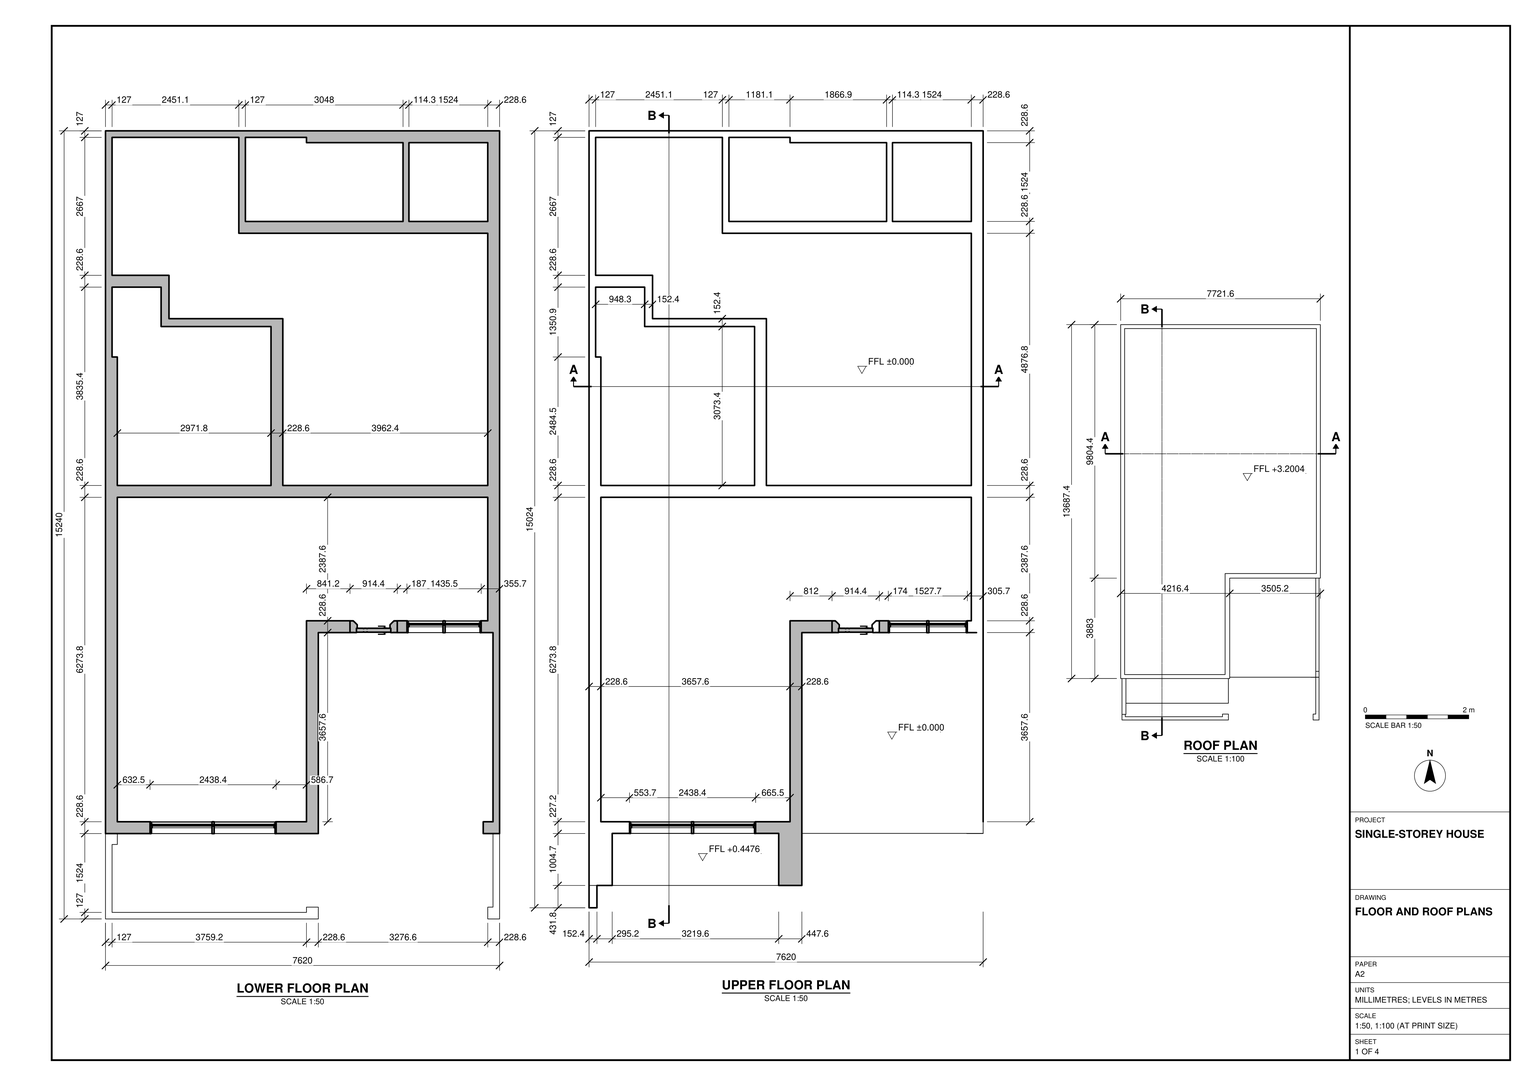
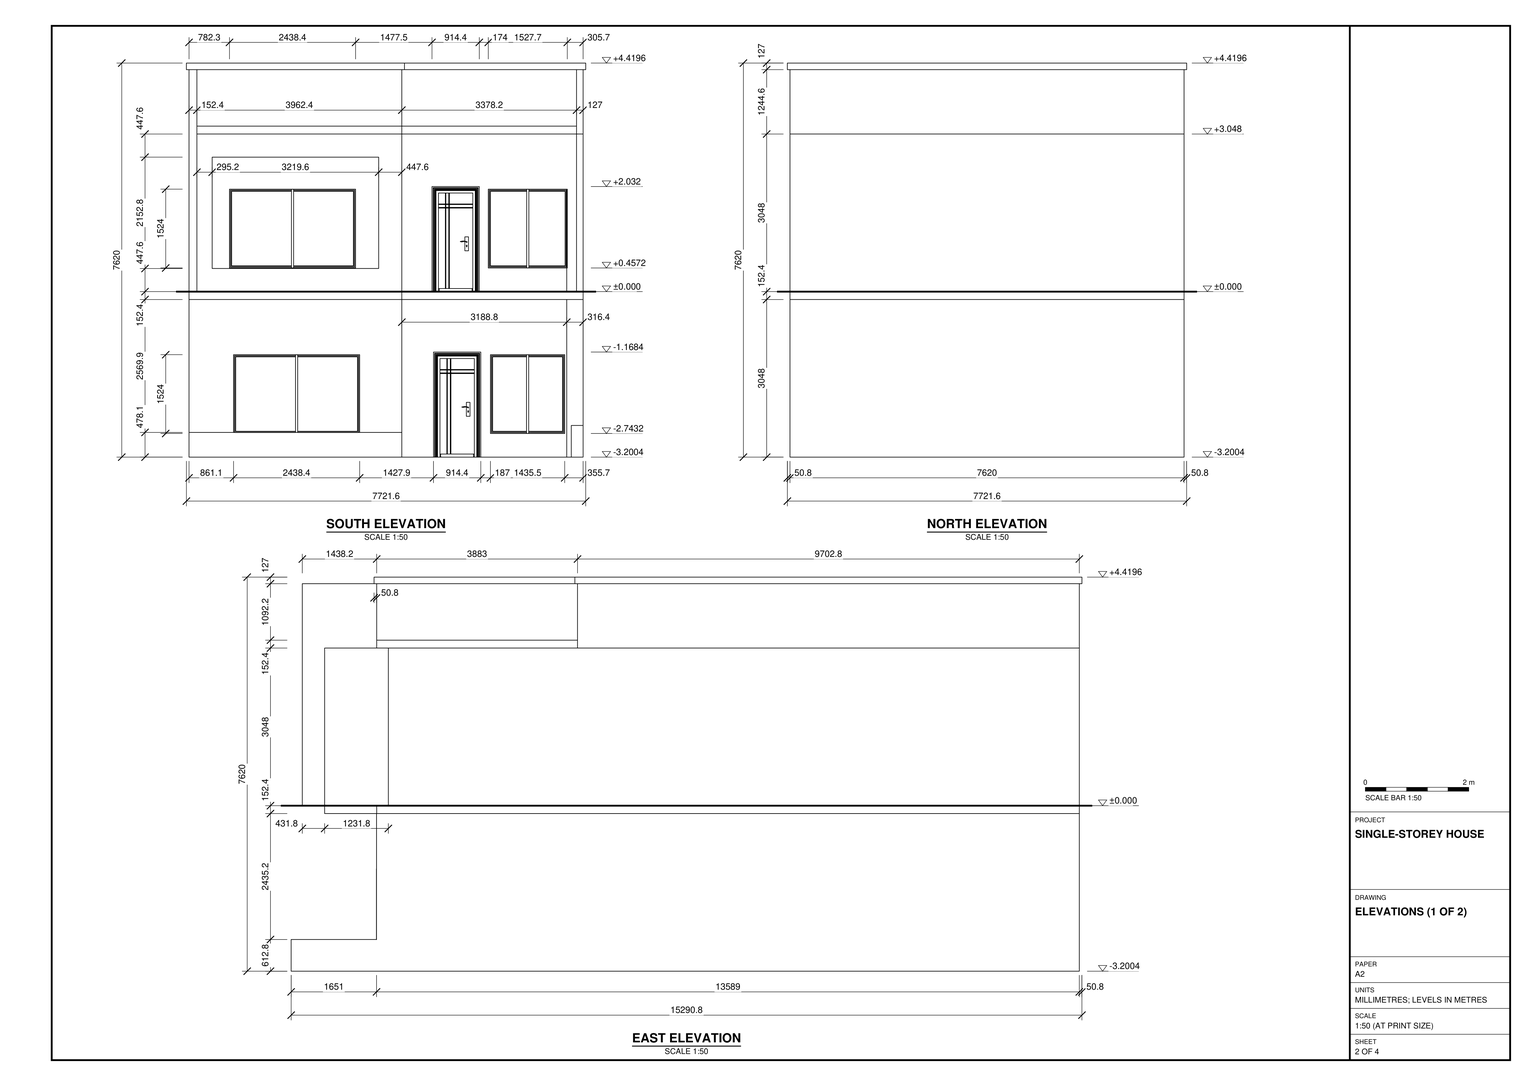
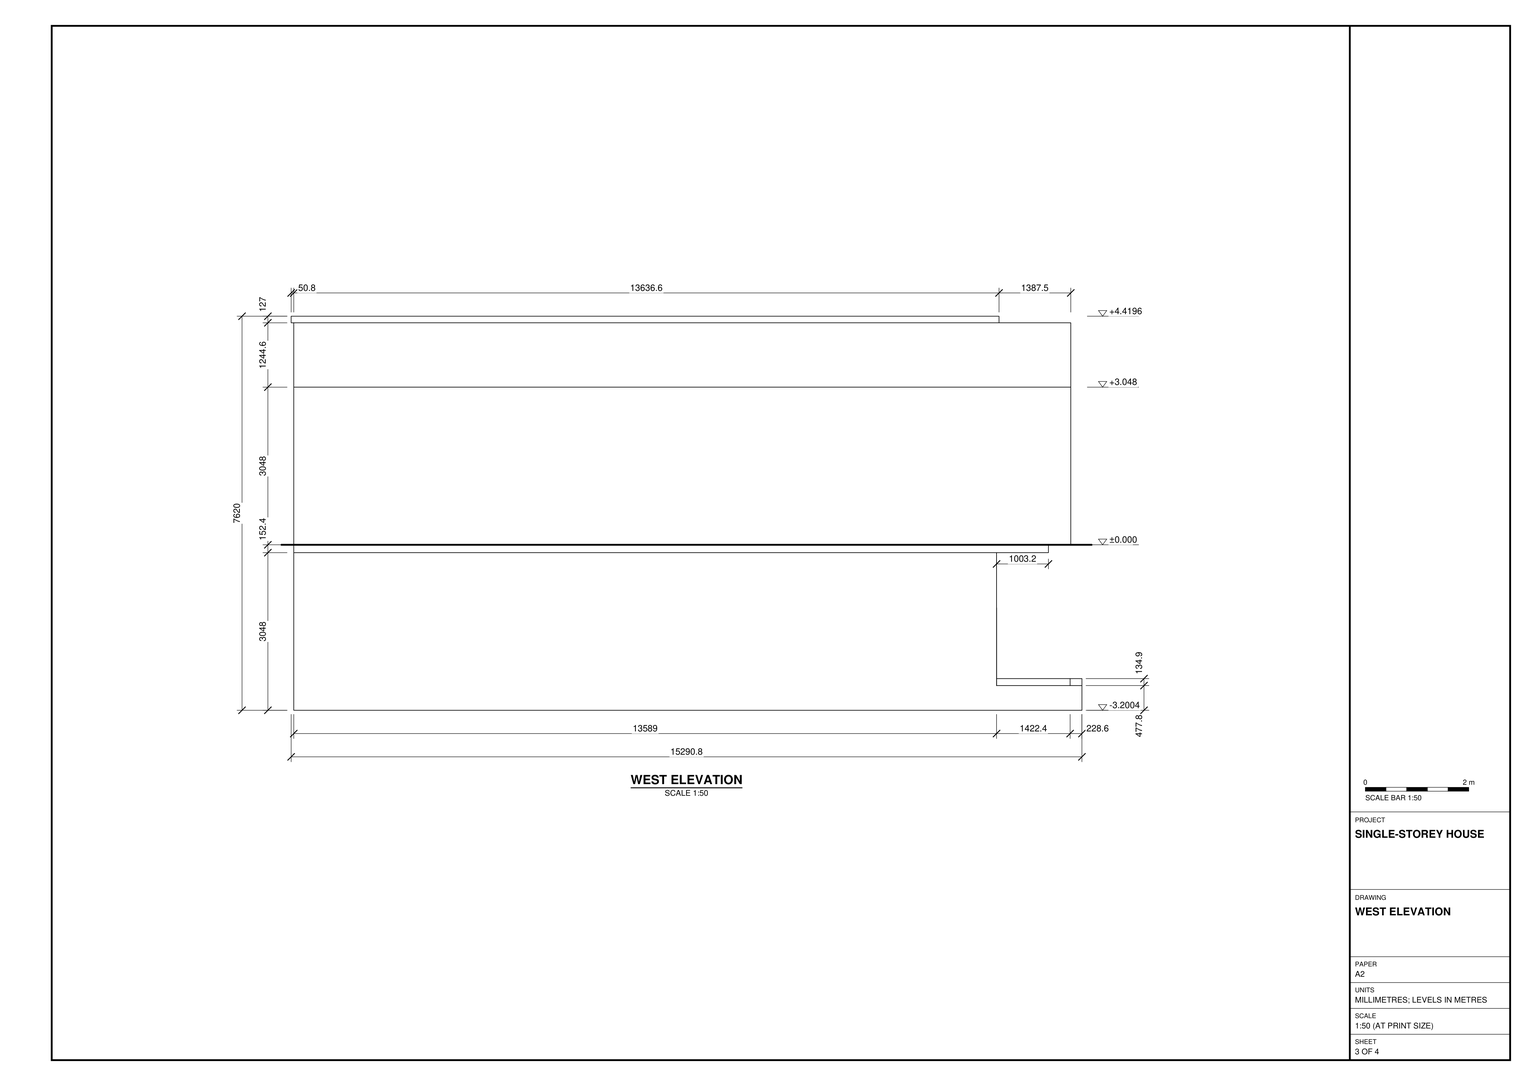
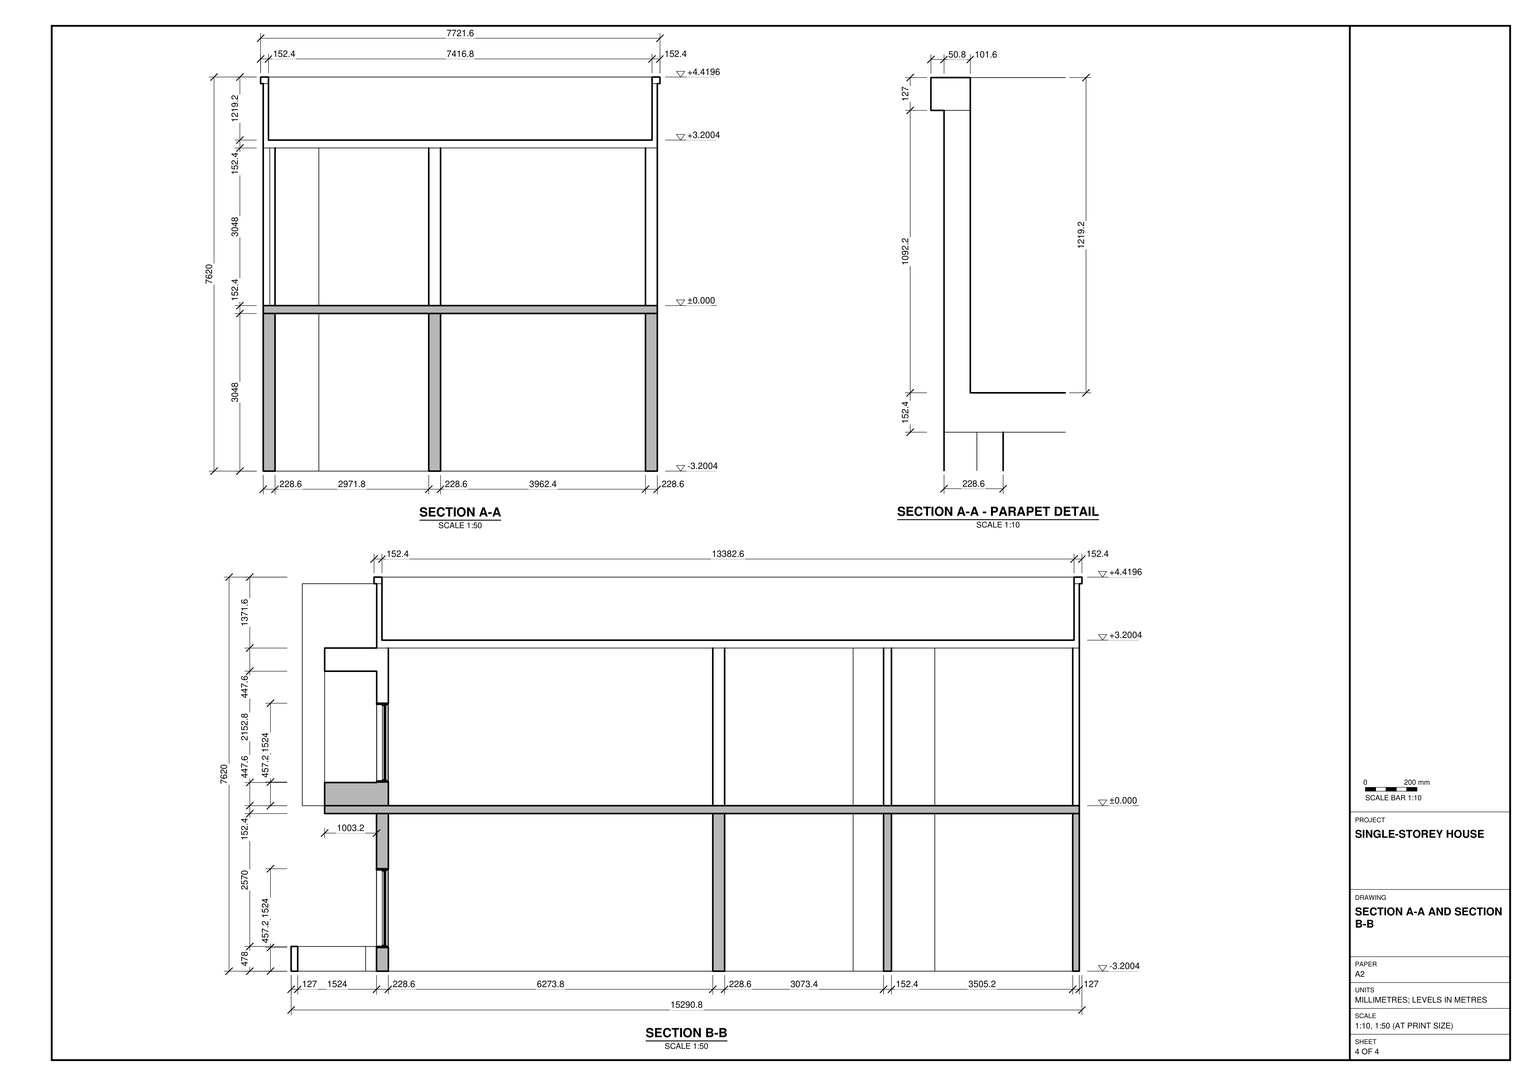
Build the house in SketchUp from task_files/diagram_01.pdf. Work in millimetres, with X running east–west and Y running north–south. The overall dimensions are 7721.6 mm wide, 15290.8 mm deep and 7620 mm high. Use the upper floor at 0 mm as the reference datum. The lower floor is at −3200.4 mm and the top of the roof edge is at +4419.6 mm.

Follow the lower and upper plans separately. At the south end, project the wide window bay forward on the west and set the entrance wall back on the east. Include the low walls and slab edges that extend beyond the enclosed rooms. Lay out the full-width cross wall, the stepped partition on the west and the smaller compartments at the north end. Use the wall thickness dimensioned for each run rather than one thickness throughout.

Fit the framed doors and divided windows on the south elevation. Keep the north, east and west faces closed as drawn. Match the flat roof to its stepped plan and show its narrow projecting cap. Keep walls, slabs, roof and any furniture or joinery pieces in separate groups or components, and use components for repeated parts. Any decor or loose items shown may be represented by suitable library components. Save one SketchUp model as output_files/flat_roofed_house_with_a_stepped_south_frontage.skp.

# SketchUp Ruby script. Lengths in millimetres.
U = 1.mm
M = Sketchup.active_model
def pt(a) = Geom::Point3d.new(a.map { |v| v * U })
def face(e, loops, mat)
  f = e.add_face(loops[0].map { |a| pt(a) })
  loops[1..].each { |l| e.add_face(l.map { |a| pt(a) }).erase! }
  f.material = f.back_material = mat if mat
  f
end
# faces: each face lists its corners as indices into pts; further lists are holes
def faces(e, pts, list, mat = nil) = list.each { |f| face(e, (f[0].is_a?(Array) ? f : [f]).map { |l| l.map { |i| pts[i] } }, mat) }
# xy, xz, yz: faces in a plane at the given z, y or x. An outline is a flat list of corners, or four numbers for a rectangle; further outlines are holes
def ring(l) = l.size == 4 ? [[l[0], l[1]], [l[2], l[1]], [l[2], l[3]], [l[0], l[3]]] : l.each_slice(2).to_a
def flat(e, list, mat, &to3) = list.each { |f| face(e, (f[0].is_a?(Array) ? f : [f]).map { |l| ring(l).map { |u, v| to3.(u, v) } }, mat) }
def xy(e, z, list, mat = nil) = flat(e, list, mat) { |x, y| [x, y, z] }
def xz(e, y, list, mat = nil) = flat(e, list, mat) { |x, z| [x, y, z] }
def yz(e, x, list, mat = nil) = flat(e, list, mat) { |y, z| [x, y, z] }
def lines(e, pts, list) = list.each { |a, b| e.add_line(pt(pts[a]), pt(pts[b])) }
# prism: a flat outline (further loops are holes) pulled along v
def prism(e, loops, v, mat = nil)
  f = face(e, loops, mat); d = Geom::Vector3d.new(v.map { |x| x * U })
  f.pushpull(f.normal.samedirection?(d) ? d.length : -d.length)
end
def box(e, o, s, mat = nil) = prism(e, [[o, [o[0] + s[0], o[1], o[2]], [o[0] + s[0], o[1] + s[1], o[2]], [o[0], o[1] + s[1], o[2]]]], [0, 0, s[2]], mat)
def at(x, y, z, deg = 0) = Geom::Transformation.translation(pt([x, y, z])) * Geom::Transformation.rotation(ORIGIN, Z_AXIS, deg.degrees)
def axes(o, x, y, z) = Geom::Transformation.new([*x, 0, *y, 0, *z, 0, *pt(o).to_a, 1])
def part(name) = M.definitions.add(name)
# library, detail: a bought-in or finely detailed component or shape, given as its bounding box
def library(name, o, s) = part(name).tap { |d| box(d.entities, o, s) }
def detail(e, o, s) = box(e.add_group.entities, o, s)
def put(e, d, t, mat = nil) = e.add_instance(d, t).tap { |i| i.material = mat if mat }
def group(e, t, mat = nil) = e.add_group.tap { |g| g.transformation = t; g.material = mat if mat }.entities
root = M.entities
M.materials.add("[Metal Silver]").color = [234, 233, 238]
M.materials.add("[Translucent Glass Blue]").color = [100, 149, 237]
M.materials["[Translucent Glass Blue]"].alpha = 0.5
M.materials.add("[Wax 01]").color = [250, 213, 163]
c1 = library("Group\#5",[0,0,0],[914.4,266,2032])
c2 = part("Group12\#2")
box(c2.entities,[26,54.1,26],[2386.4,16,1472])
c3 = library("Group\#6",[0,0,0],[914.4,266,2032])
c4 = part("Group19\#2")
box(c4.entities,[26,54.9,26],[2386.4,16,1472])
c5 = part("Group22\#2")
box(c5.entities,[26,54.9,26],[1475.7,16,1472])
c6 = part("Group25\#2")
box(c6.entities,[26,54.9,26],[1383.4,16,1472])
xy(root,0,[[[50.8,0,50.8,15240,7670.8,15240,7670.8,0,7442.2,0,7442.2,228.6,7543.8,228.6,7543.8,1651,7354.4,1651,7354.4,1879.6,7543.8,1879.6,7543.8,5537.2,5692.6,5537.2,5692.6,5765.8,7442.2,5765.8,7442.2,8153.4,279.4,8153.4,279.4,1879.6,3937,1879.6,3937,5765.8,4778.2,5765.8,4778.2,5537.2,4165.6,5537.2,4165.6,1651,279.4,1651,279.4,1440.1,177.8,1440.1,177.8,127,3937,127,3937,228.6,4165.6,228.6,4165.6,0],[3479.8,8382,7442.2,8382,7442.2,13258.8,2628.9,13258.8,2628.9,15113,177.8,15113,177.8,12446,1278.5,12446,1278.5,11607.8,3479.8,11607.8],[279.4,8382,3251.2,8382,3251.2,11455.4,1126.1,11455.4,1126.1,12217.4,177.8,12217.4,177.8,10866.5,279.4,10866.5],[2755.9,13487.4,5803.9,13487.4,5803.9,15011.4,3937,15011.4,3937,15113,2755.9,15113],[5918.2,13487.4,7442.2,15011.4]]])
xy(root,457.2,[[911.9,1651,3350.3,1879.6],[5879.6,5537.2,7315.1,5765.8]])
xy(root,477.8,[[50.8,0,4165.6,0,4165.6,228.6,3937,228.6,3937,127,177.8,127,177.8,1440.1,279.4,1440.1,279.4,1651,50.8,1651]])
xy(root,612.8,[[7442.2,0,7670.8,0,7670.8,1651,7543.8,1651,7543.8,228.6,7442.2,228.6]])
xy(root,1981.2,[[911.9,1651,3350.3,1879.6],[5879.6,5537.2,7315.1,5765.8]])
xy(root,2032,[[4778.2,5537.2,5692.6,5765.8]])
xy(root,3048,[[[50.8,1651,4165.6,1651,4165.6,5537.2,7543.8,5537.2,7543.8,1879.6,7354.4,1879.6,7354.4,1651,7670.8,1651,7670.8,15240,50.8,15240],[279.4,1879.6,279.4,8153.4,7442.2,8153.4,7442.2,5765.8,3937,5765.8,3937,1879.6],[3479.8,8382,3479.8,11607.8,1278.5,11607.8,1278.5,12446,177.8,12446,177.8,15113,2628.9,15113,2628.9,13258.8,7442.2,13258.8,7442.2,8382],[279.4,8382,279.4,10866.5,177.8,10866.5,177.8,12217.4,1126.1,12217.4,1126.1,11455.4,3251.2,11455.4,3251.2,8382],[2755.9,13487.4,2755.9,15113,3937,15113,3937,15011.4,5803.9,15011.4,5803.9,13487.4],[5918.2,13487.4,7442.2,15011.4]]])
xz(root,0,[[50.8,0,4165.6,477.8],[7442.2,0,7670.8,612.8]])
xz(root,127,[[177.8,0,3937,477.8]])
xz(root,228.6,[[3937,0,4165.6,477.8],[7442.2,0,7543.8,612.8]])
xz(root,1440.1,[[177.8,0,279.4,477.8]])
xz(root,1651,[[[279.4,0,4165.6,0,4165.6,3048,50.8,3048,50.8,477.8,279.4,477.8],[911.9,457.2,3350.3,1981.2]],[7354.4,0,7543.8,0,7543.8,612.8,7670.8,612.8,7670.8,3048,7354.4,3048]])
xz(root,1879.6,[[[279.4,0,3937,3048],[911.9,457.2,3350.3,1981.2]],[7354.4,0,7543.8,3048]])
xz(root,5537.2,[[[4165.6,0,4778.2,0,4778.2,2032,5692.6,2032,5692.6,0,7543.8,0,7543.8,3048,4165.6,3048],[5879.6,457.2,7315.1,1981.2]]])
xz(root,5765.8,[[[3937,0,3937,3048,7442.2,3048,7442.2,0,5692.6,0,5692.6,2032,4778.2,2032,4778.2,0],[5879.6,457.2,7315.1,1981.2]]])
xz(root,8153.4,[[279.4,0,7442.2,3048]])
xz(root,8382,[[279.4,0,3251.2,3048],[3479.8,0,7442.2,3048]])
xz(root,10866.5,[[177.8,0,279.4,3048]])
xz(root,11455.4,[[1126.1,0,3251.2,3048]])
xz(root,11607.8,[[1278.5,0,3479.8,3048]])
xz(root,12217.4,[[177.8,0,1126.1,3048]])
xz(root,12446,[[177.8,0,1278.5,3048]])
xz(root,13258.8,[[2628.9,0,7442.2,3048]])
xz(root,13487.4,[[2755.9,0,5803.9,3048],[5918.2,0,7442.2,3048]])
xz(root,15011.4,[[3937,0,5803.9,3048],[5918.2,0,7442.2,3048]])
xz(root,15113,[[177.8,0,2628.9,3048],[2755.9,0,3937,3048]])
xz(root,15240,[[50.8,0,7670.8,3048]])
yz(root,50.8,[[0,0,0,477.8,1651,477.8,1651,3048,15240,3048,15240,0]])
yz(root,177.8,[[127,0,1440.1,477.8],[10866.5,0,12217.4,3048],[12446,0,15113,3048]])
yz(root,279.4,[[1440.1,0,1651,477.8],[1879.6,0,8153.4,3048],[8382,0,10866.5,3048]])
yz(root,911.9,[[1651,457.2,1879.6,1981.2]])
yz(root,1126.1,[[11455.4,0,12217.4,3048]])
yz(root,1278.5,[[11607.8,0,12446,3048]])
yz(root,2628.9,[[13258.8,0,15113,3048]])
yz(root,2755.9,[[13487.4,0,15113,3048]])
yz(root,3251.2,[[8382,0,11455.4,3048]])
yz(root,3350.3,[[1651,457.2,1879.6,1981.2]])
yz(root,3479.8,[[8382,0,11607.8,3048]])
yz(root,3937,[[127,0,228.6,477.8],[1879.6,0,5765.8,3048],[15011.4,0,15113,3048]])
yz(root,4165.6,[[0,0,228.6,477.8],[1651,0,5537.2,3048]])
yz(root,4778.2,[[5537.2,0,5765.8,2032]])
yz(root,5692.6,[[5537.2,0,5765.8,2032]])
yz(root,5803.9,[[13487.4,0,15011.4,3048]])
yz(root,5879.6,[[5537.2,457.2,5765.8,1981.2]])
yz(root,5918.2,[[13487.4,0,15011.4,3048]])
yz(root,7315.1,[[5537.2,457.2,5765.8,1981.2]])
yz(root,7354.4,[[1651,0,1879.6,3048]])
yz(root,7442.2,[[0,0,228.6,612.8],[5765.8,0,8153.4,3048],[8382,0,13258.8,3048],[13487.4,0,15011.4,3048]])
yz(root,7543.8,[[228.6,0,1651,612.8],[1879.6,0,5537.2,3048]])
yz(root,7670.8,[[0,0,15240,0,15240,3048,1651,3048,1651,612.8,0,612.8]])
p = [[949.3,1651,481.9],[949.3,1879.6,481.9],[949.3,1651,2128.2],[949.3,1879.6,2128.2],[3535.4,1651,481.9],[3535.4,1879.6,481.9],
  [3535.4,1651,2128.2],[3535.4,1879.6,2128.2],[4165.6,1649.2,1980.2],[4165.6,1651,1980.2],[7543.8,1654.2,6248.4],[7354.4,1654.2,6248.4],
  [7354.4,5537.2,6248.4],[7543.8,5537.2,6248.4]]
lines(root,p,[[0,1],[2,3],[4,5],[6,7],[8,9],[10,11],[11,12],[12,13],[13,10]])
g1 = group(root,at(50.8,1654.2,3048))
prism(g1,[[[7620,13585.8,0],[7620,0,0],[4114.8,0,0],[4114.8,-1006.5,0],[0,-1006.5,0],[0,13585.8,0]]],[0,0,152.4])
g2 = group(root,at(0,1603.4,3200.4),"[Wax 01]")
xy(g2,447.6,[[498.4,-955.7,3718,50.8]],"[Wax 01]")
xy(g2,457.2,[[833.1,50.8,3271.5,276.2],[5837.4,3933.8,7365.1,4162.4]])
xy(g2,1981.2,[[833.1,50.8,3271.5,276.2],[5837.4,3933.8,7365.1,4162.4]])
xy(g2,2032,[[4749,3933.8,5663.4,4162.4]])
xy(g2,2600.4,[[498.4,-955.7,3718,50.8]],"[Wax 01]")
xy(g2,3048,[[203.2,-955.7,4165.6,50.8],[4165.6,50.8,7354.4,3933.8],[7354.4,50.8,7543.8,3933.8],[7543.8,276.2,7670.8,3933.8]])
xy(g2,3200.4,[[4165.6,50.8,7543.8,3933.8],[152.4,152.4,4038.6,152.4,4038.6,4060.8,7569.2,4060.8,7569.2,13535,152.4,13535]])
xy(g2,4292.6,[[50.8,-1387.5,203.2,0],[0,0,50.8,50.8],[203.2,0,4216.4,50.8],[0,50.8,50.8,13636.6],[4165.6,50.8,4216.4,152.4],
  [4165.6,152.4,4165.6,3933.8,7721.6,3933.8,7721.6,3883,4216.4,3883,4216.4,152.4],[7670.8,3933.8,7721.6,13687.4],[0,13636.6,7670.8,13687.4]])
xy(g2,4419.6,[[[0,0,4216.4,0,4216.4,3883,7721.6,3883,7721.6,13687.4,0,13687.4],[152.4,152.4,152.4,13535,7569.2,13535,7569.2,4060.8,4038.6,4060.8,4038.6,152.4]]])
xz(g2,-1387.5,[[50.8,0,203.2,4292.6]])
xz(g2,-955.7,[[[203.2,0,4165.6,3048],[498.4,447.6,3718,2600.4]]],"[Wax 01]")
xz(g2,0,[[0,4292.6,4216.4,4419.6]])
xz(g2,50.8,[[203.2,3048,4165.6,3200.4],[4165.6,3048,7543.8,3200.4],[203.2,3200.4,4165.6,4292.6]])
xz(g2,50.8,[[[498.4,447.6,3718,2600.4],[833.1,457.2,3271.5,1981.2]]],"[Wax 01]")
xz(g2,152.4,[[152.4,3200.4,4038.6,4419.6]])
xz(g2,276.2,[[[279.4,0,3937,3048],[833.1,457.2,3271.5,1981.2]]])
xz(g2,3883,[[4216.4,4292.6,7721.6,4419.6]])
xz(g2,3933.8,[[7354.4,457.2,7365.1,1981.2],[7543.8,3048,7670.8,4292.6],[4165.6,3200.4,7543.8,4292.6]])
xz(g2,3933.8,[[4165.6,0,4749,0,4749,2032,5663.4,2032,5663.4,0,7354.4,0,7354.4,457.2,5837.4,457.2,5837.4,1981.2,7365.1,1981.2,7365.1,457.2,7354.4,457.2,7354.4,0,7543.8,0,7543.8,3048,4165.6,3048]],"[Wax 01]")
xz(g2,4060.8,[[4038.6,3200.4,7569.2,4419.6]])
xz(g2,4162.4,[[[3937,0,3937,3048,7442.2,3048,7442.2,0,5663.4,0,5663.4,2032,4749,2032,4749,0],[5837.4,457.2,7365.1,1981.2]]])
xz(g2,6550,[[279.4,0,7442.2,3048]])
xz(g2,6778.6,[[279.4,0,3251.2,3048],[3479.8,0,7442.2,3048]])
xz(g2,9263.1,[[177.8,0,279.4,3048]])
xz(g2,9852,[[1126.1,0,3251.2,3048]])
xz(g2,10004.4,[[1278.5,0,3479.8,3048]])
xz(g2,10614,[[177.8,0,1126.1,3048]])
xz(g2,10842.6,[[177.8,0,1278.5,3048]])
xz(g2,11655.4,[[2628.9,0,7442.2,3048]])
xz(g2,11884,[[2755.9,0,5803.9,3048],[5918.2,0,7442.2,3048]])
xz(g2,13408,[[3937,0,5803.9,3048],[5918.2,0,7442.2,3048]])
xz(g2,13509.6,[[177.8,0,2628.9,3048],[2755.9,0,3937,3048]])
xz(g2,13535,[[152.4,3200.4,7569.2,4419.6]])
xz(g2,13636.6,[[50.8,0,7670.8,3048],[50.8,3048,7670.8,4292.6]])
xz(g2,13687.4,[[0,4292.6,7721.6,4419.6]])
yz(g2,0,[[0,4292.6,13687.4,4419.6]])
yz(g2,50.8,[[-1387.5,0,13636.6,3048],[-1387.5,3048,13636.6,4292.6]])
yz(g2,152.4,[[152.4,3200.4,13535,4419.6]])
yz(g2,177.8,[[9263.1,0,10614,3048],[10842.6,0,13509.6,3048]])
yz(g2,203.2,[[-1387.5,0,-955.7,0,-955.7,3048,50.8,3048,50.8,4292.6,-1387.5,4292.6]])
yz(g2,279.4,[[276.2,0,6550,3048],[6778.6,0,9263.1,3048]])
yz(g2,498.4,[[-955.7,447.6,50.8,2600.4]],"[Wax 01]")
yz(g2,833.1,[[50.8,457.2,276.2,1981.2]])
yz(g2,1126.1,[[9852,0,10614,3048]])
yz(g2,1278.5,[[10004.4,0,10842.6,3048]])
yz(g2,2628.9,[[11655.4,0,13509.6,3048]])
yz(g2,2755.9,[[11884,0,13509.6,3048]])
yz(g2,3251.2,[[6778.6,0,9852,3048]])
yz(g2,3271.5,[[50.8,457.2,276.2,1981.2]])
yz(g2,3479.8,[[6778.6,0,10004.4,3048]])
yz(g2,3718,[[-955.7,447.6,50.8,2600.4]],"[Wax 01]")
yz(g2,3937,[[276.2,0,4162.4,3048],[13408,0,13509.6,3048]])
yz(g2,4038.6,[[152.4,3200.4,3933.8,4419.6],[3933.8,3200.4,4060.8,4419.6]])
yz(g2,4165.6,[[50.8,3200.4,3933.8,4292.6]])
yz(g2,4165.6,[[-955.7,0,3933.8,3048]],"[Wax 01]")
yz(g2,4216.4,[[0,4292.6,3883,4419.6]])
yz(g2,4749,[[3933.8,0,4162.4,2032]])
yz(g2,5663.4,[[3933.8,0,4162.4,2032]])
yz(g2,5803.9,[[11884,0,13408,3048]])
yz(g2,5837.4,[[3933.8,457.2,4162.4,1981.2]])
yz(g2,5918.2,[[11884,0,13408,3048]])
yz(g2,7365.1,[[3933.8,457.2,4162.4,1981.2]])
yz(g2,7442.2,[[4162.4,0,6550,3048],[6778.6,0,11655.4,3048],[11884,0,13408,3048]])
yz(g2,7543.8,[[50.8,3048,3933.8,3200.4]])
yz(g2,7569.2,[[4060.8,3200.4,13535,4419.6]])
yz(g2,7670.8,[[276.2,0,13636.6,3048],[3933.8,3048,13636.6,4292.6]])
yz(g2,7721.6,[[3883,4292.6,13687.4,4419.6]])
put(g2,c1,at(4749,3896.4,0))
g3 = group(g2,at(3271.5,276.2,457.2,180))
g4 = group(g3,at(0,0,0),"[Metal Silver]")
xy(g4,0,[[0,0,1198.2,225.4],[1198.2,0,1240.2,225.4],[1240.2,0,2438.4,225.4]])
xy(g4,21,[[21,115.4,1198.2,223.6],[1240.2,115.4,2417.4,223.6]])
xy(g4,26,[[26,54.1,1198.2,82.9],[1198.2,54.1,1240.2,82.9],[1240.2,54.1,2412.4,82.9]])
xy(g4,41,[[41,45.1,1198.2,54.1],[1240.2,45.1,2397.4,54.1]])
xy(g4,42,[[42,82.9,1198.2,86.5],[1240.2,82.9,2396.4,86.5]])
xy(g4,1482,[[42,82.9,1198.2,86.5],[1240.2,82.9,2396.4,86.5]])
xy(g4,1483,[[41,45.1,1198.2,54.1],[1240.2,45.1,2397.4,54.1]])
xy(g4,1498,[[26,54.1,1198.2,82.9],[1198.2,54.1,1240.2,82.9],[1240.2,54.1,2412.4,82.9]])
xy(g4,1503,[[21,115.4,1198.2,223.6],[1240.2,115.4,2417.4,223.6]])
xy(g4,1524,[[0,0,1198.2,225.4],[1198.2,0,1240.2,225.4],[1240.2,0,2438.4,225.4]])
xz(g4,0,[[0,0,1198.2,0,1198.2,10,10,10,10,1514,1198.2,1514,1198.2,1524,0,1524],[1198.2,0,1240.2,1524],[1240.2,0,2438.4,0,2438.4,1524,1240.2,1524,1240.2,1514,2428.4,1514,2428.4,10,1240.2,10]])
xz(g4,9,[[15,15,1198.2,15,1198.2,20,20,20,20,1504,1198.2,1504,1198.2,1509,15,1509],[1240.2,15,2423.4,15,2423.4,1509,1240.2,1509,1240.2,1504,2418.4,1504,2418.4,20,1240.2,20]])
xz(g4,45.1,[[21,21,1198.2,21,1198.2,41,41,41,41,1483,1198.2,1483,1198.2,1503,21,1503],[1240.2,21,2417.4,21,2417.4,1503,1240.2,1503,1240.2,1483,2397.4,1483,2397.4,41,1240.2,41]])
xz(g4,54.1,[[26,26,26,1498,1198.2,1498,1198.2,1483,41,1483,41,41,1198.2,41,1198.2,26],[1198.2,26,1240.2,1498],[1240.2,26,1240.2,41,2397.4,41,2397.4,1483,1240.2,1483,1240.2,1498,2412.4,1498,2412.4,26]])
xz(g4,82.9,[[26,26,1198.2,26,1198.2,42,42,42,42,1482,1198.2,1482,1198.2,1498,26,1498],[1198.2,26,1240.2,1498],[1240.2,26,2412.4,26,2412.4,1498,1240.2,1498,1240.2,1482,2396.4,1482,2396.4,42,1240.2,42]])
xz(g4,115.4,[[21,21,21,1503,1198.2,1503,1198.2,1486,38,1486,38,38,1198.2,38,1198.2,21],[1240.2,21,1240.2,38,2400.4,38,2400.4,1486,1240.2,1486,1240.2,1503,2417.4,1503,2417.4,21]])
xz(g4,227.2,[[1,1,1,1523,1198.2,1523,1198.2,1505,19,1505,19,19,1198.2,19,1198.2,1],[1198.2,1,1240.2,1523],[1240.2,1,1240.2,19,2419.4,19,2419.4,1505,1240.2,1505,1240.2,1523,2437.4,1523,2437.4,1]])
yz(g4,0,[[0,0,225.4,1524]])
yz(g4,21,[[115.4,21,223.6,1503]])
yz(g4,26,[[54.1,26,82.9,1498]])
yz(g4,41,[[45.1,41,54.1,1483]])
yz(g4,42,[[82.9,42,86.5,1482]])
yz(g4,1198.2,[[0,0,225.4,0,227.2,1,227.2,19,223.6,21,115.4,21,115.4,38,86.5,42,82.9,42,82.9,26,54.1,26,54.1,41,45.1,41,45.1,21,9,20,9,15,0,10],[[0,0,0,1524,225.4,1524,227.2,1523,227.2,1,225.4,0],[54.1,26,82.9,1498]],[82.9,1482,86.5,1482,115.4,1486,115.4,1503,223.6,1503,227.2,1505,227.2,1523,225.4,1524,0,1524,0,1514,9,1509,9,1504,45.1,1503,45.1,1483,54.1,1483,54.1,1498,82.9,1498]])
yz(g4,1240.2,[[0,0,0,10,9,15,9,20,45.1,21,45.1,41,54.1,41,54.1,26,82.9,26,82.9,42,86.5,42,115.4,38,115.4,21,223.6,21,227.2,19,227.2,1,225.4,0],[[0,0,225.4,0,227.2,1,227.2,1523,225.4,1524,0,1524],[54.1,26,82.9,1498]],[82.9,1482,82.9,1498,54.1,1498,54.1,1483,45.1,1483,45.1,1503,9,1504,9,1509,0,1514,0,1524,225.4,1524,227.2,1523,227.2,1505,223.6,1503,115.4,1503,115.4,1486,86.5,1482]])
yz(g4,2396.4,[[82.9,42,86.5,1482]])
yz(g4,2397.4,[[45.1,41,54.1,1483]])
yz(g4,2412.4,[[54.1,26,82.9,1498]])
yz(g4,2417.4,[[115.4,21,223.6,1503]])
yz(g4,2438.4,[[0,0,225.4,1524]])
p = [[1198.2,227.2,1],[1198.2,225.4,0],[0,225.4,0],[1,227.2,1],[0,225.4,1524],[1,227.2,1523],
  [1240.2,227.2,1],[1240.2,225.4,0],[2437.4,227.2,1],[2438.4,225.4,0],[2437.4,227.2,1523],[2438.4,225.4,1524],
  [1198.2,0,10],[1198.2,9,15],[15,9,15],[10,0,10],[15,9,1509],[10,0,1514],
  [1240.2,9,15],[1240.2,0,10],[2428.4,0,10],[2423.4,9,15],[2428.4,0,1514],[2423.4,9,1509],
  [1198.2,223.6,21],[1198.2,227.2,19],[19,227.2,19],[21,223.6,21],[19,227.2,1505],[21,223.6,1503],
  [1240.2,227.2,19],[1240.2,223.6,21],[2417.4,223.6,21],[2419.4,227.2,19],[2417.4,223.6,1503],[2419.4,227.2,1505],
  [1198.2,9,20],[1198.2,45.1,21],[21,45.1,21],[20,9,20],[21,45.1,1503],[20,9,1504],
  [1240.2,45.1,21],[1240.2,9,20],[2418.4,9,20],[2417.4,45.1,21],[2418.4,9,1504],[2417.4,45.1,1503],
  [1198.2,86.5,42],[1198.2,115.4,38],[38,115.4,38],[42,86.5,42],[38,115.4,1486],[42,86.5,1482],
  [1240.2,115.4,38],[1240.2,86.5,42],[2396.4,86.5,42],[2400.4,115.4,38],[2396.4,86.5,1482],[2400.4,115.4,1486],
  [1198.2,115.4,1486],[1198.2,86.5,1482],[1240.2,86.5,1482],[1240.2,115.4,1486],[1198.2,45.1,1503],[1198.2,9,1504],
  [1240.2,9,1504],[1240.2,45.1,1503],[1198.2,227.2,1505],[1198.2,223.6,1503],[1240.2,223.6,1503],[1240.2,227.2,1505],
  [1198.2,9,1509],[1198.2,0,1514],[1240.2,0,1514],[1240.2,9,1509],[1198.2,225.4,1524],[1198.2,227.2,1523],
  [1240.2,225.4,1524],[1240.2,227.2,1523]]
faces(g4,p,[[0,1,2,3],[3,2,4,5],[1,0,6,7],[7,6,8,9],[9,8,10,11],[12,13,14,15],[15,14,16,17],[18,19,20,21],
  [21,20,22,23],[24,25,26,27],[27,26,28,29],[30,31,32,33],[33,32,34,35],[36,37,38,39],[39,38,40,41],[42,43,44,45],
  [45,44,46,47],[48,49,50,51],[51,50,52,53],[54,55,56,57],[57,56,58,59],[53,52,60,61],[59,58,62,63],[41,40,64,65],
  [47,46,66,67],[29,28,68,69],[35,34,70,71],[17,16,72,73],[23,22,74,75],[5,4,76,77],[77,76,78,79],[11,10,79,78]])
put(g3,c2,at(0,0,0),"[Translucent Glass Blue]")
put(root,c3,at(4778.2,5499.8,0))
g5 = group(root,at(3350.3,1879.6,457.2,180))
put(g5,c4,at(0,0,0),"[Translucent Glass Blue]")
g6 = group(g5,at(0,0,0),"[Metal Silver]")
xy(g6,0,[[0,0,1198.2,228.6],[1198.2,0,1240.2,228.6],[1240.2,0,2438.4,228.6]])
xy(g6,21,[[21,117,1198.2,226.8],[1240.2,117,2417.4,226.8]])
xy(g6,26,[[26,54.9,1198.2,84.1],[1198.2,54.9,1240.2,84.1],[1240.2,54.9,2412.4,84.1]])
xy(g6,41,[[41,45.7,1198.2,54.9],[1240.2,45.7,2397.4,54.9]])
xy(g6,42,[[42,84.1,1198.2,87.8],[1240.2,84.1,2396.4,87.8]])
xy(g6,1482,[[42,84.1,1198.2,87.8],[1240.2,84.1,2396.4,87.8]])
xy(g6,1483,[[41,45.7,1198.2,54.9],[1240.2,45.7,2397.4,54.9]])
xy(g6,1498,[[26,54.9,1198.2,84.1],[1198.2,54.9,1240.2,84.1],[1240.2,54.9,2412.4,84.1]])
xy(g6,1503,[[21,117,1198.2,226.8],[1240.2,117,2417.4,226.8]])
xy(g6,1524,[[0,0,1198.2,228.6],[1198.2,0,1240.2,228.6],[1240.2,0,2438.4,228.6]])
xz(g6,0,[[0,0,1198.2,0,1198.2,10,10,10,10,1514,1198.2,1514,1198.2,1524,0,1524],[1198.2,0,1240.2,1524],[1240.2,0,2438.4,0,2438.4,1524,1240.2,1524,1240.2,1514,2428.4,1514,2428.4,10,1240.2,10]])
xz(g6,9.1,[[15,15,1198.2,15,1198.2,20,20,20,20,1504,1198.2,1504,1198.2,1509,15,1509],[1240.2,15,2423.4,15,2423.4,1509,1240.2,1509,1240.2,1504,2418.4,1504,2418.4,20,1240.2,20]])
xz(g6,45.7,[[21,21,1198.2,21,1198.2,41,41,41,41,1483,1198.2,1483,1198.2,1503,21,1503],[1240.2,21,2417.4,21,2417.4,1503,1240.2,1503,1240.2,1483,2397.4,1483,2397.4,41,1240.2,41]])
xz(g6,54.9,[[26,26,26,1498,1198.2,1498,1198.2,1483,41,1483,41,41,1198.2,41,1198.2,26],[1198.2,26,1240.2,1498],[1240.2,26,1240.2,41,2397.4,41,2397.4,1483,1240.2,1483,1240.2,1498,2412.4,1498,2412.4,26]])
xz(g6,84.1,[[26,26,1198.2,26,1198.2,42,42,42,42,1482,1198.2,1482,1198.2,1498,26,1498],[1198.2,26,1240.2,1498],[1240.2,26,2412.4,26,2412.4,1498,1240.2,1498,1240.2,1482,2396.4,1482,2396.4,42,1240.2,42]])
xz(g6,117,[[21,21,21,1503,1198.2,1503,1198.2,1486,38,1486,38,38,1198.2,38,1198.2,21],[1240.2,21,1240.2,38,2400.4,38,2400.4,1486,1240.2,1486,1240.2,1503,2417.4,1503,2417.4,21]])
xz(g6,230.4,[[1,1,1,1523,1198.2,1523,1198.2,1505,19,1505,19,19,1198.2,19,1198.2,1],[1198.2,1,1240.2,1523],[1240.2,1,1240.2,19,2419.4,19,2419.4,1505,1240.2,1505,1240.2,1523,2437.4,1523,2437.4,1]])
yz(g6,0,[[0,0,228.6,1524]])
yz(g6,21,[[117,21,226.8,1503]])
yz(g6,26,[[54.9,26,84.1,1498]])
yz(g6,41,[[45.7,41,54.9,1483]])
yz(g6,42,[[84.1,42,87.8,1482]])
yz(g6,1198.2,[[0,0,228.6,0,230.4,1,230.4,19,226.8,21,117,21,117,38,87.8,42,84.1,42,84.1,26,54.9,26,54.9,41,45.7,41,45.7,21,9.1,20,9.1,15,0,10],[[0,0,0,1524,228.6,1524,230.4,1523,230.4,1,228.6,0],[54.9,26,84.1,1498]],[84.1,1482,87.8,1482,117,1486,117,1503,226.8,1503,230.4,1505,230.4,1523,228.6,1524,0,1524,0,1514,9.1,1509,9.1,1504,45.7,1503,45.7,1483,54.9,1483,54.9,1498,84.1,1498]])
yz(g6,1240.2,[[0,0,0,10,9.1,15,9.1,20,45.7,21,45.7,41,54.9,41,54.9,26,84.1,26,84.1,42,87.8,42,117,38,117,21,226.8,21,230.4,19,230.4,1,228.6,0],[[0,0,228.6,0,230.4,1,230.4,1523,228.6,1524,0,1524],[54.9,26,84.1,1498]],[84.1,1482,84.1,1498,54.9,1498,54.9,1483,45.7,1483,45.7,1503,9.1,1504,9.1,1509,0,1514,0,1524,228.6,1524,230.4,1523,230.4,1505,226.8,1503,117,1503,117,1486,87.8,1482]])
yz(g6,2396.4,[[84.1,42,87.8,1482]])
yz(g6,2397.4,[[45.7,41,54.9,1483]])
yz(g6,2412.4,[[54.9,26,84.1,1498]])
yz(g6,2417.4,[[117,21,226.8,1503]])
yz(g6,2438.4,[[0,0,228.6,1524]])
p = [[1198.2,230.4,1],[1198.2,228.6,0],[0,228.6,0],[1,230.4,1],[0,228.6,1524],[1,230.4,1523],
  [1240.2,230.4,1],[1240.2,228.6,0],[2437.4,230.4,1],[2438.4,228.6,0],[2437.4,230.4,1523],[2438.4,228.6,1524],
  [1198.2,0,10],[1198.2,9.1,15],[15,9.1,15],[10,0,10],[15,9.1,1509],[10,0,1514],
  [1240.2,9.1,15],[1240.2,0,10],[2428.4,0,10],[2423.4,9.1,15],[2428.4,0,1514],[2423.4,9.1,1509],
  [1198.2,226.8,21],[1198.2,230.4,19],[19,230.4,19],[21,226.8,21],[19,230.4,1505],[21,226.8,1503],
  [1240.2,230.4,19],[1240.2,226.8,21],[2417.4,226.8,21],[2419.4,230.4,19],[2417.4,226.8,1503],[2419.4,230.4,1505],
  [1198.2,9.1,20],[1198.2,45.7,21],[21,45.7,21],[20,9.1,20],[21,45.7,1503],[20,9.1,1504],
  [1240.2,45.7,21],[1240.2,9.1,20],[2418.4,9.1,20],[2417.4,45.7,21],[2418.4,9.1,1504],[2417.4,45.7,1503],
  [1198.2,87.8,42],[1198.2,117,38],[38,117,38],[42,87.8,42],[38,117,1486],[42,87.8,1482],
  [1240.2,117,38],[1240.2,87.8,42],[2396.4,87.8,42],[2400.4,117,38],[2396.4,87.8,1482],[2400.4,117,1486],
  [1198.2,117,1486],[1198.2,87.8,1482],[1240.2,87.8,1482],[1240.2,117,1486],[1198.2,45.7,1503],[1198.2,9.1,1504],
  [1240.2,9.1,1504],[1240.2,45.7,1503],[1198.2,230.4,1505],[1198.2,226.8,1503],[1240.2,226.8,1503],[1240.2,230.4,1505],
  [1198.2,9.1,1509],[1198.2,0,1514],[1240.2,0,1514],[1240.2,9.1,1509],[1198.2,228.6,1524],[1198.2,230.4,1523],
  [1240.2,228.6,1524],[1240.2,230.4,1523]]
faces(g6,p,[[0,1,2,3],[3,2,4,5],[1,0,6,7],[7,6,8,9],[9,8,10,11],[12,13,14,15],[15,14,16,17],[18,19,20,21],
  [21,20,22,23],[24,25,26,27],[27,26,28,29],[30,31,32,33],[33,32,34,35],[36,37,38,39],[39,38,40,41],[42,43,44,45],
  [45,44,46,47],[48,49,50,51],[51,50,52,53],[54,55,56,57],[57,56,58,59],[53,52,60,61],[59,58,62,63],[41,40,64,65],
  [47,46,66,67],[29,28,68,69],[35,34,70,71],[17,16,72,73],[23,22,74,75],[5,4,76,77],[77,76,78,79],[11,10,79,78]])
g7 = group(root,at(7365.1,5765.8,3657.6,180))
g8 = group(g7,at(0,0,0),"[Metal Silver]")
xy(g8,0,[[0,0,742.9,228.6],[742.9,0,784.9,228.6],[784.9,0,1527.7,228.6]])
xy(g8,21,[[21,117,742.9,226.8],[784.9,117,1506.7,226.8]])
xy(g8,26,[[26,54.9,742.9,84.1],[742.9,54.9,784.9,84.1],[784.9,54.9,1501.7,84.1]])
xy(g8,41,[[41,45.7,742.9,54.9],[784.9,45.7,1486.7,54.9]])
xy(g8,42,[[42,84.1,742.9,87.8],[784.9,84.1,1485.7,87.8]])
xy(g8,1482,[[42,84.1,742.9,87.8],[784.9,84.1,1485.7,87.8]])
xy(g8,1483,[[41,45.7,742.9,54.9],[784.9,45.7,1486.7,54.9]])
xy(g8,1498,[[26,54.9,742.9,84.1],[742.9,54.9,784.9,84.1],[784.9,54.9,1501.7,84.1]])
xy(g8,1503,[[21,117,742.9,226.8],[784.9,117,1506.7,226.8]])
xy(g8,1524,[[0,0,742.9,228.6],[742.9,0,784.9,228.6],[784.9,0,1527.7,228.6]])
xz(g8,0,[[0,0,742.9,0,742.9,10,10,10,10,1514,742.9,1514,742.9,1524,0,1524],[742.9,0,784.9,1524],[784.9,0,1527.7,0,1527.7,1524,784.9,1524,784.9,1514,1517.7,1514,1517.7,10,784.9,10]])
xz(g8,9.1,[[15,15,742.9,15,742.9,20,20,20,20,1504,742.9,1504,742.9,1509,15,1509],[784.9,15,1512.7,15,1512.7,1509,784.9,1509,784.9,1504,1507.7,1504,1507.7,20,784.9,20]])
xz(g8,45.7,[[21,21,742.9,21,742.9,41,41,41,41,1483,742.9,1483,742.9,1503,21,1503],[784.9,21,1506.7,21,1506.7,1503,784.9,1503,784.9,1483,1486.7,1483,1486.7,41,784.9,41]])
xz(g8,54.9,[[26,26,26,1498,742.9,1498,742.9,1483,41,1483,41,41,742.9,41,742.9,26],[742.9,26,784.9,1498],[784.9,26,784.9,41,1486.7,41,1486.7,1483,784.9,1483,784.9,1498,1501.7,1498,1501.7,26]])
xz(g8,84.1,[[26,26,742.9,26,742.9,42,42,42,42,1482,742.9,1482,742.9,1498,26,1498],[742.9,26,784.9,1498],[784.9,26,1501.7,26,1501.7,1498,784.9,1498,784.9,1482,1485.7,1482,1485.7,42,784.9,42]])
xz(g8,117,[[21,21,21,1503,742.9,1503,742.9,1486,38,1486,38,38,742.9,38,742.9,21],[784.9,21,784.9,38,1489.7,38,1489.7,1486,784.9,1486,784.9,1503,1506.7,1503,1506.7,21]])
xz(g8,230.4,[[1,1,1,1523,742.9,1523,742.9,1505,19,1505,19,19,742.9,19,742.9,1],[742.9,1,784.9,1523],[784.9,1,784.9,19,1508.7,19,1508.7,1505,784.9,1505,784.9,1523,1526.7,1523,1526.7,1]])
yz(g8,0,[[0,0,228.6,1524]])
yz(g8,21,[[117,21,226.8,1503]])
yz(g8,26,[[54.9,26,84.1,1498]])
yz(g8,41,[[45.7,41,54.9,1483]])
yz(g8,42,[[84.1,42,87.8,1482]])
yz(g8,742.9,[[0,0,228.6,0,230.4,1,230.4,19,226.8,21,117,21,117,38,87.8,42,84.1,42,84.1,26,54.9,26,54.9,41,45.7,41,45.7,21,9.1,20,9.1,15,0,10],[[0,0,0,1524,228.6,1524,230.4,1523,230.4,1,228.6,0],[54.9,26,84.1,1498]],[84.1,1482,87.8,1482,117,1486,117,1503,226.8,1503,230.4,1505,230.4,1523,228.6,1524,0,1524,0,1514,9.1,1509,9.1,1504,45.7,1503,45.7,1483,54.9,1483,54.9,1498,84.1,1498]])
yz(g8,784.9,[[0,0,0,10,9.1,15,9.1,20,45.7,21,45.7,41,54.9,41,54.9,26,84.1,26,84.1,42,87.8,42,117,38,117,21,226.8,21,230.4,19,230.4,1,228.6,0],[[0,0,228.6,0,230.4,1,230.4,1523,228.6,1524,0,1524],[54.9,26,84.1,1498]],[84.1,1482,84.1,1498,54.9,1498,54.9,1483,45.7,1483,45.7,1503,9.1,1504,9.1,1509,0,1514,0,1524,228.6,1524,230.4,1523,230.4,1505,226.8,1503,117,1503,117,1486,87.8,1482]])
yz(g8,1485.7,[[84.1,42,87.8,1482]])
yz(g8,1486.7,[[45.7,41,54.9,1483]])
yz(g8,1501.7,[[54.9,26,84.1,1498]])
yz(g8,1506.7,[[117,21,226.8,1503]])
yz(g8,1527.7,[[0,0,228.6,1524]])
p = [[742.9,230.4,1],[742.9,228.6,0],[0,228.6,0],[1,230.4,1],[0,228.6,1524],[1,230.4,1523],
  [784.9,230.4,1],[784.9,228.6,0],[1526.7,230.4,1],[1527.7,228.6,0],[1526.7,230.4,1523],[1527.7,228.6,1524],
  [742.9,0,10],[742.9,9.1,15],[15,9.1,15],[10,0,10],[15,9.1,1509],[10,0,1514],
  [784.9,9.1,15],[784.9,0,10],[1517.7,0,10],[1512.7,9.1,15],[1517.7,0,1514],[1512.7,9.1,1509],
  [742.9,226.8,21],[742.9,230.4,19],[19,230.4,19],[21,226.8,21],[19,230.4,1505],[21,226.8,1503],
  [784.9,230.4,19],[784.9,226.8,21],[1506.7,226.8,21],[1508.7,230.4,19],[1506.7,226.8,1503],[1508.7,230.4,1505],
  [742.9,9.1,20],[742.9,45.7,21],[21,45.7,21],[20,9.1,20],[21,45.7,1503],[20,9.1,1504],
  [784.9,45.7,21],[784.9,9.1,20],[1507.7,9.1,20],[1506.7,45.7,21],[1507.7,9.1,1504],[1506.7,45.7,1503],
  [742.9,87.8,42],[742.9,117,38],[38,117,38],[42,87.8,42],[38,117,1486],[42,87.8,1482],
  [784.9,117,38],[784.9,87.8,42],[1485.7,87.8,42],[1489.7,117,38],[1485.7,87.8,1482],[1489.7,117,1486],
  [742.9,117,1486],[742.9,87.8,1482],[784.9,87.8,1482],[784.9,117,1486],[742.9,45.7,1503],[742.9,9.1,1504],
  [784.9,9.1,1504],[784.9,45.7,1503],[742.9,230.4,1505],[742.9,226.8,1503],[784.9,226.8,1503],[784.9,230.4,1505],
  [742.9,9.1,1509],[742.9,0,1514],[784.9,0,1514],[784.9,9.1,1509],[742.9,228.6,1524],[742.9,230.4,1523],
  [784.9,228.6,1524],[784.9,230.4,1523]]
faces(g8,p,[[0,1,2,3],[3,2,4,5],[1,0,6,7],[7,6,8,9],[9,8,10,11],[12,13,14,15],[15,14,16,17],[18,19,20,21],
  [21,20,22,23],[24,25,26,27],[27,26,28,29],[30,31,32,33],[33,32,34,35],[36,37,38,39],[39,38,40,41],[42,43,44,45],
  [45,44,46,47],[48,49,50,51],[51,50,52,53],[54,55,56,57],[57,56,58,59],[53,52,60,61],[59,58,62,63],[41,40,64,65],
  [47,46,66,67],[29,28,68,69],[35,34,70,71],[17,16,72,73],[23,22,74,75],[5,4,76,77],[77,76,78,79],[11,10,79,78]])
put(g7,c5,at(0,0,0),"[Translucent Glass Blue]")
g9 = group(root,at(7315.1,5765.8,457.2,180))
g10 = group(g9,at(0,0,0),"[Metal Silver]")
xy(g10,0,[[0,0,696.7,228.6],[696.7,0,738.7,228.6],[738.7,0,1435.4,228.6]])
xy(g10,21,[[21,117,696.7,226.8],[738.7,117,1414.4,226.8]])
xy(g10,26,[[26,54.9,696.7,84.1],[696.7,54.9,738.7,84.1],[738.7,54.9,1409.4,84.1]])
xy(g10,41,[[41,45.7,696.7,54.9],[738.7,45.7,1394.4,54.9]])
xy(g10,42,[[42,84.1,696.7,87.8],[738.7,84.1,1393.4,87.8]])
xy(g10,1482,[[42,84.1,696.7,87.8],[738.7,84.1,1393.4,87.8]])
xy(g10,1483,[[41,45.7,696.7,54.9],[738.7,45.7,1394.4,54.9]])
xy(g10,1498,[[26,54.9,696.7,84.1],[696.7,54.9,738.7,84.1],[738.7,54.9,1409.4,84.1]])
xy(g10,1503,[[21,117,696.7,226.8],[738.7,117,1414.4,226.8]])
xy(g10,1524,[[0,0,696.7,228.6],[696.7,0,738.7,228.6],[738.7,0,1435.4,228.6]])
xz(g10,0,[[0,0,696.7,0,696.7,10,10,10,10,1514,696.7,1514,696.7,1524,0,1524],[696.7,0,738.7,1524],[738.7,0,1435.4,0,1435.4,1524,738.7,1524,738.7,1514,1425.4,1514,1425.4,10,738.7,10]])
xz(g10,9.1,[[15,15,696.7,15,696.7,20,20,20,20,1504,696.7,1504,696.7,1509,15,1509],[738.7,15,1420.4,15,1420.4,1509,738.7,1509,738.7,1504,1415.4,1504,1415.4,20,738.7,20]])
xz(g10,45.7,[[21,21,696.7,21,696.7,41,41,41,41,1483,696.7,1483,696.7,1503,21,1503],[738.7,21,1414.4,21,1414.4,1503,738.7,1503,738.7,1483,1394.4,1483,1394.4,41,738.7,41]])
xz(g10,54.9,[[26,26,26,1498,696.7,1498,696.7,1483,41,1483,41,41,696.7,41,696.7,26],[696.7,26,738.7,1498],[738.7,26,738.7,41,1394.4,41,1394.4,1483,738.7,1483,738.7,1498,1409.4,1498,1409.4,26]])
xz(g10,84.1,[[26,26,696.7,26,696.7,42,42,42,42,1482,696.7,1482,696.7,1498,26,1498],[696.7,26,738.7,1498],[738.7,26,1409.4,26,1409.4,1498,738.7,1498,738.7,1482,1393.4,1482,1393.4,42,738.7,42]])
xz(g10,117,[[21,21,21,1503,696.7,1503,696.7,1486,38,1486,38,38,696.7,38,696.7,21],[738.7,21,738.7,38,1397.4,38,1397.4,1486,738.7,1486,738.7,1503,1414.4,1503,1414.4,21]])
xz(g10,230.4,[[1,1,1,1523,696.7,1523,696.7,1505,19,1505,19,19,696.7,19,696.7,1],[696.7,1,738.7,1523],[738.7,1,738.7,19,1416.4,19,1416.4,1505,738.7,1505,738.7,1523,1434.4,1523,1434.4,1]])
yz(g10,0,[[0,0,228.6,1524]])
yz(g10,21,[[117,21,226.8,1503]])
yz(g10,26,[[54.9,26,84.1,1498]])
yz(g10,41,[[45.7,41,54.9,1483]])
yz(g10,42,[[84.1,42,87.8,1482]])
yz(g10,696.7,[[0,0,228.6,0,230.4,1,230.4,19,226.8,21,117,21,117,38,87.8,42,84.1,42,84.1,26,54.9,26,54.9,41,45.7,41,45.7,21,9.1,20,9.1,15,0,10],[[0,0,0,1524,228.6,1524,230.4,1523,230.4,1,228.6,0],[54.9,26,84.1,1498]],[84.1,1482,87.8,1482,117,1486,117,1503,226.8,1503,230.4,1505,230.4,1523,228.6,1524,0,1524,0,1514,9.1,1509,9.1,1504,45.7,1503,45.7,1483,54.9,1483,54.9,1498,84.1,1498]])
yz(g10,738.7,[[0,0,0,10,9.1,15,9.1,20,45.7,21,45.7,41,54.9,41,54.9,26,84.1,26,84.1,42,87.8,42,117,38,117,21,226.8,21,230.4,19,230.4,1,228.6,0],[[0,0,228.6,0,230.4,1,230.4,1523,228.6,1524,0,1524],[54.9,26,84.1,1498]],[84.1,1482,84.1,1498,54.9,1498,54.9,1483,45.7,1483,45.7,1503,9.1,1504,9.1,1509,0,1514,0,1524,228.6,1524,230.4,1523,230.4,1505,226.8,1503,117,1503,117,1486,87.8,1482]])
yz(g10,1393.4,[[84.1,42,87.8,1482]])
yz(g10,1394.4,[[45.7,41,54.9,1483]])
yz(g10,1409.4,[[54.9,26,84.1,1498]])
yz(g10,1414.4,[[117,21,226.8,1503]])
yz(g10,1435.4,[[0,0,228.6,1524]])
p = [[696.7,230.4,1],[696.7,228.6,0],[0,228.6,0],[1,230.4,1],[0,228.6,1524],[1,230.4,1523],
  [738.7,230.4,1],[738.7,228.6,0],[1434.4,230.4,1],[1435.4,228.6,0],[1434.4,230.4,1523],[1435.4,228.6,1524],
  [696.7,0,10],[696.7,9.1,15],[15,9.1,15],[10,0,10],[15,9.1,1509],[10,0,1514],
  [738.7,9.1,15],[738.7,0,10],[1425.4,0,10],[1420.4,9.1,15],[1425.4,0,1514],[1420.4,9.1,1509],
  [696.7,226.8,21],[696.7,230.4,19],[19,230.4,19],[21,226.8,21],[19,230.4,1505],[21,226.8,1503],
  [738.7,230.4,19],[738.7,226.8,21],[1414.4,226.8,21],[1416.4,230.4,19],[1414.4,226.8,1503],[1416.4,230.4,1505],
  [696.7,9.1,20],[696.7,45.7,21],[21,45.7,21],[20,9.1,20],[21,45.7,1503],[20,9.1,1504],
  [738.7,45.7,21],[738.7,9.1,20],[1415.4,9.1,20],[1414.4,45.7,21],[1415.4,9.1,1504],[1414.4,45.7,1503],
  [696.7,87.8,42],[696.7,117,38],[38,117,38],[42,87.8,42],[38,117,1486],[42,87.8,1482],
  [738.7,117,38],[738.7,87.8,42],[1393.4,87.8,42],[1397.4,117,38],[1393.4,87.8,1482],[1397.4,117,1486],
  [696.7,117,1486],[696.7,87.8,1482],[738.7,87.8,1482],[738.7,117,1486],[696.7,45.7,1503],[696.7,9.1,1504],
  [738.7,9.1,1504],[738.7,45.7,1503],[696.7,230.4,1505],[696.7,226.8,1503],[738.7,226.8,1503],[738.7,230.4,1505],
  [696.7,9.1,1509],[696.7,0,1514],[738.7,0,1514],[738.7,9.1,1509],[696.7,228.6,1524],[696.7,230.4,1523],
  [738.7,228.6,1524],[738.7,230.4,1523]]
faces(g10,p,[[0,1,2,3],[3,2,4,5],[1,0,6,7],[7,6,8,9],[9,8,10,11],[12,13,14,15],[15,14,16,17],[18,19,20,21],
  [21,20,22,23],[24,25,26,27],[27,26,28,29],[30,31,32,33],[33,32,34,35],[36,37,38,39],[39,38,40,41],[42,43,44,45],
  [45,44,46,47],[48,49,50,51],[51,50,52,53],[54,55,56,57],[57,56,58,59],[53,52,60,61],[59,58,62,63],[41,40,64,65],
  [47,46,66,67],[29,28,68,69],[35,34,70,71],[17,16,72,73],[23,22,74,75],[5,4,76,77],[77,76,78,79],[11,10,79,78]])
put(g9,c6,at(0,0,0),"[Translucent Glass Blue]")
